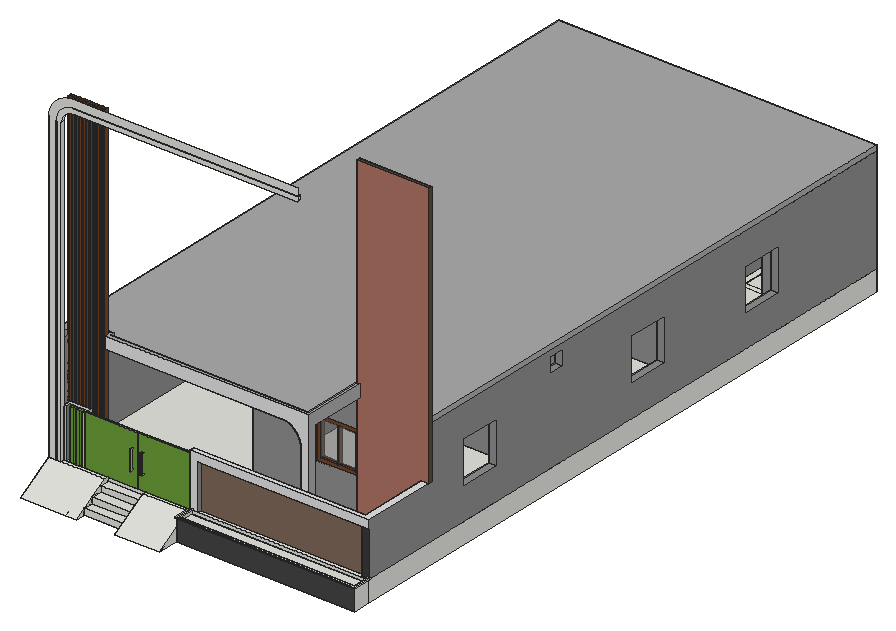
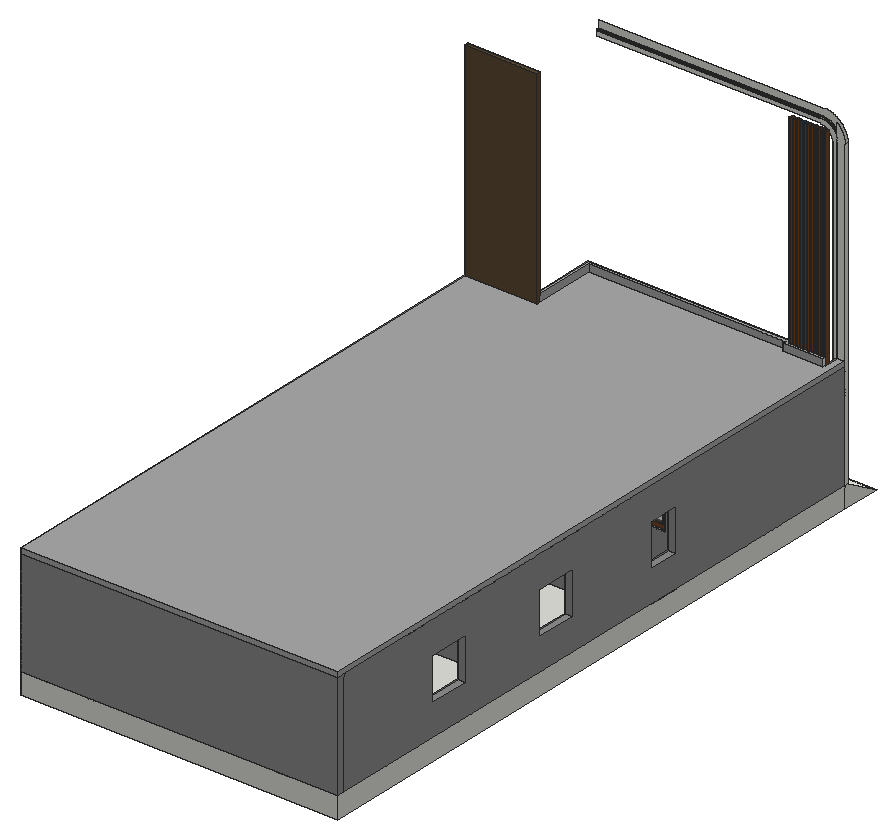
# SketchUp Ruby script. Lengths in inches.
U = 1.inch
M = Sketchup.active_model
def pt(a) = Geom::Point3d.new(a.map { |v| v * U })
def face(e, loops, mat)
  f = e.add_face(loops[0].map { |a| pt(a) })
  loops[1..].each { |l| e.add_face(l.map { |a| pt(a) }).erase! }
  f.material = f.back_material = mat if mat
  f
end
# faces: each face lists its corners as indices into pts; further lists are holes
def faces(e, pts, list, mat = nil) = list.each { |f| face(e, (f[0].is_a?(Array) ? f : [f]).map { |l| l.map { |i| pts[i] } }, mat) }
# xy, xz, yz: faces in a plane at the given z, y or x. An outline is a flat list of corners, or four numbers for a rectangle; further outlines are holes
def ring(l) = l.size == 4 ? [[l[0], l[1]], [l[2], l[1]], [l[2], l[3]], [l[0], l[3]]] : l.each_slice(2).to_a
def flat(e, list, mat, &to3) = list.each { |f| face(e, (f[0].is_a?(Array) ? f : [f]).map { |l| ring(l).map { |u, v| to3.(u, v) } }, mat) }
def xy(e, z, list, mat = nil) = flat(e, list, mat) { |x, y| [x, y, z] }
def xz(e, y, list, mat = nil) = flat(e, list, mat) { |x, z| [x, y, z] }
def yz(e, x, list, mat = nil) = flat(e, list, mat) { |y, z| [x, y, z] }
def lines(e, pts, list) = list.each { |a, b| e.add_line(pt(pts[a]), pt(pts[b])) }
# prism: a flat outline (further loops are holes) pulled along v
def prism(e, loops, v, mat = nil)
  f = face(e, loops, mat); d = Geom::Vector3d.new(v.map { |x| x * U })
  f.pushpull(f.normal.samedirection?(d) ? d.length : -d.length)
end
def box(e, o, s, mat = nil) = prism(e, [[o, [o[0] + s[0], o[1], o[2]], [o[0] + s[0], o[1] + s[1], o[2]], [o[0], o[1] + s[1], o[2]]]], [0, 0, s[2]], mat)
def at(x, y, z, deg = 0) = Geom::Transformation.translation(pt([x, y, z])) * Geom::Transformation.rotation(ORIGIN, Z_AXIS, deg.degrees)
def axes(o, x, y, z) = Geom::Transformation.new([*x, 0, *y, 0, *z, 0, *pt(o).to_a, 1])
def part(name) = M.definitions.add(name)
# library, detail: a bought-in or finely detailed component or shape, given as its bounding box
def library(name, o, s) = part(name).tap { |d| box(d.entities, o, s) }
def detail(e, o, s) = box(e.add_group.entities, o, s)
def put(e, d, t, mat = nil) = e.add_instance(d, t).tap { |i| i.material = mat if mat }
def group(e, t, mat = nil) = e.add_group.tap { |g| g.transformation = t; g.material = mat if mat }.entities
root = M.entities
M.materials.add("Material5_ met").color = [196, 146, 107]
M.materials.add("[Brick Rough Dark]").color = [94, 77, 53]
M.materials.add("[Color M01]").color = [226, 226, 226]
M.materials.add("[Color M03]").color = [170, 170, 170]
M.materials.add("[Color M04]").color = [142, 142, 142]
M.materials.add("[Color M07]").color = [58, 58, 58]
M.materials.add("[Granite Brown]").color = [126, 104, 91]
M.materials.add("[Granite Dark Gray]").color = [69, 68, 68]
M.materials.add("[Grass Dark Green]").color = [106, 157, 55]
M.materials.add("[Polished Concrete New]").color = [200, 200, 203]
M.materials.add("[Stone Flagstone Ashlar]").color = [175, 116, 102]
M.materials.add("[Translucent Glass Gray]").color = [128, 128, 128]
M.materials["[Translucent Glass Gray]"].alpha = 0.5
M.materials.add("[Wood Veneer 01]").color = [120, 70, 37]
M.materials.add("polished steel").color = [183, 187, 190]
M.materials.add("polished_ Blacktop Old 01").color = [132, 136, 139]
M.materials.add("steel").color = [179, 179, 179]
c1 = part("*U6")
p = [[-20,-17,0],[-20,23,0],[-18.25,23,0],[-18.25,-17,0],[20,-17,0],[19.92,-14.49,0],
  [19.68,-11.99,0],[19.29,-9.5,0],[18.74,-7.05,0],[18.04,-4.64,0],[17.19,-2.28,0],[16.19,0.03,0],
  [15.05,2.27,0],[13.77,4.43,0],[12.36,6.51,0],[10.82,8.5,0],[9.16,10.38,0],[7.38,12.16,0],
  [5.5,13.82,0],[3.51,15.36,0],[1.43,16.77,0],[-0.73,18.05,0],[-2.97,19.19,0],[-5.28,20.19,0],
  [-7.64,21.04,0],[-10.05,21.74,0],[-12.5,22.29,0],[-14.99,22.68,0],[-17.49,22.92,0],[-20,-23,0],
  [20,-23,0]]
lines(c1.entities,p,[[0,1],[1,2],[2,3],[3,0],[4,5],[5,6],[6,7],[7,8],[8,9],[9,10],[10,11],[11,12],
  [12,13],[13,14],[14,15],[15,16],[16,17],[17,18],[18,19],[19,20],[20,21],[21,22],[22,23],[23,24],
  [24,25],[25,26],[26,27],[27,28],[28,1],[0,29],[4,30]])
c2 = part("new block 03")
p = [[-4.5,18,0],[4.5,18,0],[4.5,-18,0],[-4.5,-18,0],[-1.33,-18,0],[-1.33,18,0],
  [1.57,18,0],[1.57,-18,0]]
lines(c2.entities,p,[[0,1],[1,2],[2,3],[3,0],[4,5],[5,6],[6,7]])
c3 = part("VENTILATOR")
p = [[-4.5,8.5,0],[4.5,8.5,0],[4.5,-8.5,0],[-4.5,-8.5,0],[0.58,8.5,0],[0.58,-8.5,0],
  [0,-8.5,0],[-1.15,-8.5,0],[-0.58,-8.5,0],[-0.58,8.5,0],[-1.15,8.5,0],[0,8.5,0]]
lines(c3.entities,p,[[0,1],[1,2],[2,3],[3,0],[4,5],[6,7],[8,9],[10,11]])
c4 = part("Bed - Queen")
p = [[22,23.6,0],[16.8,23.6,0],[22,38.8,0],[1.2,38.8,0],[1.2,25.6,0],[-1.2,38.8,0],
  [-1.2,25.6,0],[-22,38.8,0],[-22,25.6,0],[30,-40,0],[-30,-40,0],[-30,40,0],
  [14.8,23.2,0],[-30,23.2,0],[-30,25.6,0],[14.8,25.6,0],[30,40,0],[30,10.4,0],
  [14.8,10.4,0]]
lines(c4.entities,p,[[0,1],[2,0],[3,2],[4,3],[5,6],[7,5],[8,7],[9,10],[10,11],[12,13],[14,15],[11,16],
  [16,9],[17,15],[18,17],[15,18]])
c5 = library("*U4",[-21.75,-41.51,0],[21,28.01,0.01])
c6 = library("SINK",[-14.49,-22.42,0],[28.98,44.84,0.01])
c7 = part("new block 02")
p = [[-4.5,24,0],[4.5,24,0],[4.5,-24,0],[-4.5,-24,0],[-0.96,24,0],[-0.96,-24,0],
  [1.12,-24,0],[1.12,24,0]]
lines(c7.entities,p,[[0,1],[1,2],[2,3],[3,0],[4,5],[5,6],[6,7]])
c8 = library("PINTU 6 YA",[0,-0.6875,0],[35.83,8.07,80.71])
c9 = part("Group14\#1")
box(c9.entities,[324.26,626,0],[6,84,120])
c10 = part("Group16\#1")
box(c10.entities,[132.26,626,0],[6,84,120])
c11 = part("Group20\#1")
box(c11.entities,[233.26,464,0],[6,156,120])
c12 = part("Group25\#1")
xy(c12.entities,0,[[312.3125,242,312.3125,265.39,318.3125,265.39,318.3125,248,402.3125,248,402.3125,242],[312.3125,289.39,318.3125,296]])
xy(c12.entities,84,[[312.3125,265.39,318.3125,289.39]])
xy(c12.entities,120,[[312.3125,242,402.3125,242,402.3125,248,318.3125,248,318.3125,296,312.3125,296]])
xz(c12.entities,242,[[312.3125,0,402.3125,120]])
xz(c12.entities,248,[[318.3125,0,402.3125,120]])
xz(c12.entities,265.39,[[312.3125,0,318.3125,84]])
xz(c12.entities,289.39,[[312.3125,0,318.3125,84]])
xz(c12.entities,296,[[312.3125,0,318.3125,120]])
yz(c12.entities,312.3125,[[242,0,242,120,296,120,296,0,289.39,0,289.39,84,265.39,84,265.39,0]])
yz(c12.entities,318.3125,[[248,0,265.39,0,265.39,84,289.39,84,289.39,0,296,0,296,120,248,120]])
yz(c12.entities,402.3125,[[242,0,248,120]])
c13 = part("Group19\#1")
xy(c13.entities,0,[[-32.0625,-20.0625,-16.92,20.0625],[-15.73,-20.0625,-0.59,20.0625],[0.59,-20.0625,15.73,20.0625],[16.92,-20.0625,32.0625,20.0625]],"[Translucent Glass Gray]")
c14 = part("Group18\#1")
prism(c14.entities,[[[36,24,0],[36,-24,0],[-36,-24,0],[-36,24,0]],[[-15.73,20.0625,0],[-15.73,-20.0625,0],[-0.59,-20.0625,0],[-0.59,20.0625,0]],[[-32.0625,20.0625,0],[-32.0625,-20.0625,0],[-16.92,-20.0625,0],[-16.92,20.0625,0]],[[0.59,20.0625,0],[0.59,-20.0625,0],[15.73,-20.0625,0],[15.73,20.0625,0]],[[32.0625,20.0625,0],[16.92,20.0625,0],[16.92,-20.0625,0],[32.0625,-20.0625,0]]],[0,0,4],"[Wood Veneer 01]")
put(c14.entities,c13,at(0,0,2))
c15 = part("Group21\#2")
xy(c15.entities,0,[[-20.0625,-20.0625,-0.59,20.0625],[0.59,-20.0625,20.0625,20.0625]])
c16 = part("Group20\#3")
prism(c16.entities,[[[-24,24,0],[24,24,0],[24,-24,0],[-24,-24,0]],[[-20.0625,-20.0625,0],[-0.59,-20.0625,0],[-0.59,20.0625,0],[-20.0625,20.0625,0]],[[20.0625,20.0625,0],[0.59,20.0625,0],[0.59,-20.0625,0],[20.0625,-20.0625,0]]],[0,0,4],"[Wood Veneer 01]")
put(c16.entities,c15,at(0,0,2),"[Translucent Glass Gray]")
c17 = part("Group35\#1")
xy(c17.entities,0,[[-20.12,-20.0625,-0.59,20.0625],[0.59,-20.0625,20.12,20.0625]])
c18 = part("Group34\#2")
prism(c18.entities,[[[24.05,24,0],[24.05,-24,0],[-24.05,-24,0],[-24.05,24,0]],[[0.59,-20.0625,0],[20.12,-20.0625,0],[20.12,20.0625,0],[0.59,20.0625,0]],[[-20.12,-20.0625,0],[-0.59,-20.0625,0],[-0.59,20.0625,0],[-20.12,20.0625,0]]],[0,0,4],"[Wood Veneer 01]")
put(c18.entities,c17,at(0,0,2),"[Translucent Glass Gray]")
c19 = part("Union")
xy(c19.entities,0,[[273.03,12,282.03,21]])
xy(c19.entities,120,[[0,0,0,719,360.05,719,360.05,89,280.03,89,280.03,85,282.03,85,282.03,21,254.15,21,254.15,12,51,12,51,16,9,16,9,0]])
xy(c19.entities,126,[[0,0,9,0,9,20,55,20,55,16,278.03,16,278.03,85,280.03,85,280.03,89,360.05,89,360.05,719,0,719]])
xy(c19.entities,134,[[51,12,282.03,12,282.03,85,278.03,85,278.03,16,55,16,55,20,9,20,9,16,51,16]])
xz(c19.entities,0,[[0,120,9,126]])
xz(c19.entities,12,[[273.03,0,282.03,0,282.03,134,51,134,51,120,254.15,120,254.78,119.94,255.41,119.81,256.03,119.65,256.64,119.48,257.25,119.29,257.85,119.09,258.45,118.87,259.04,118.63,259.625,118.375,260.2,118.1,260.77,117.82,261.33,117.51,261.88,117.19,262.43,116.86,262.96,116.51,263.48,116.15,264,115.77,264.5,115.38,264.99,114.97,265.47,114.55,265.9375,114.12,266.39,113.68,266.84,113.22,267.27,112.75,268.09,111.77,268.48,111.27,268.85,110.75,269.21,110.23,269.56,109.69,269.89,109.14,270.2,108.59,270.5,108.03,270.78,107.46,271.05,106.88,271.3,106.29,271.54,105.7,271.76,105.1,271.96,104.5,272.14,103.89,272.31,103.27,272.46,102.65,272.59,102.03,272.71,101.4,272.8,100.77,272.88,100.14,272.95,99.51,272.99,98.87,273.02,98.23,273.03,97.6]],"[Color M01]")
xz(c19.entities,16,[[55,126,278.03,134]])
xz(c19.entities,16,[[9,120,51,126],[9,126,51,134]],"[Color M01]")
xz(c19.entities,20,[[9,126,55,134]])
xz(c19.entities,21,[[273.03,0,273.03,97.6,273.02,98.23,272.99,98.87,272.95,99.51,272.88,100.14,272.8,100.77,272.71,101.4,272.59,102.03,272.46,102.65,272.31,103.27,272.14,103.89,271.96,104.5,271.76,105.1,271.54,105.7,271.3,106.29,271.05,106.88,270.78,107.46,270.5,108.03,270.2,108.59,269.89,109.14,269.56,109.69,269.21,110.23,268.85,110.75,268.48,111.27,268.09,111.77,267.27,112.75,266.84,113.22,266.39,113.68,265.9375,114.12,265.47,114.55,264.99,114.97,264.5,115.38,264,115.77,263.48,116.15,262.96,116.51,262.43,116.86,261.88,117.19,261.33,117.51,260.77,117.82,260.2,118.1,259.625,118.375,259.04,118.63,258.45,118.87,257.85,119.09,257.25,119.29,256.64,119.48,256.03,119.65,255.41,119.81,254.78,119.94,254.15,120,282.03,120,282.03,0]])
xz(c19.entities,85,[[280.03,120,282.03,126],[278.03,126,282.03,134]])
xz(c19.entities,89,[[280.03,120,360.05,126]])
xz(c19.entities,719,[[0,120,360.05,126]])
yz(c19.entities,0,[[0,120,719,126]])
yz(c19.entities,9,[[0,120,16,126]])
yz(c19.entities,9,[[16,126,20,134]],"[Color M01]")
yz(c19.entities,51,[[12,120,16,134]],"[Color M01]")
yz(c19.entities,55,[[16,126,20,134]])
yz(c19.entities,273.03,[[12,0,21,97.6]])
yz(c19.entities,278.03,[[16,126,85,134]])
yz(c19.entities,280.03,[[85,120,89,126]])
yz(c19.entities,282.03,[[12,0,21,0,21,120,85,120,85,134,12,134]])
yz(c19.entities,360.05,[[89,120,719,126]])
p = [[273.03,12,97.6],[273.02,12,98.23],[273.02,21,98.23],[273.03,21,97.6],[272.99,12,98.87],[272.99,21,98.87],
  [272.95,12,99.51],[272.95,21,99.51],[272.88,12,100.14],[272.88,21,100.14],[272.8,12,100.77],[272.8,21,100.77],
  [272.71,12,101.4],[272.71,21,101.4],[272.59,12,102.03],[272.59,21,102.03],[272.46,12,102.65],[272.46,21,102.65],
  [272.31,12,103.27],[272.31,21,103.27],[272.14,12,103.89],[272.14,21,103.89],[271.96,12,104.5],[271.96,21,104.5],
  [271.76,12,105.1],[271.76,21,105.1],[271.54,12,105.7],[271.54,21,105.7],[271.3,12,106.29],[271.3,21,106.29],
  [271.05,12,106.88],[271.05,21,106.88],[270.78,12,107.46],[270.78,21,107.46],[270.5,12,108.03],[270.5,21,108.03],
  [270.2,12,108.59],[270.2,21,108.59],[269.89,12,109.14],[269.89,21,109.14],[269.56,12,109.69],[269.56,21,109.69],
  [269.21,12,110.23],[269.21,21,110.23],[268.85,12,110.75],[268.85,21,110.75],[268.48,12,111.27],[268.48,21,111.27],
  [268.09,12,111.77],[268.09,21,111.77],[267.68,12,112.26],[267.68,21,112.26],[267.27,12,112.75],[267.27,21,112.75],
  [266.84,12,113.22],[266.84,21,113.22],[266.39,12,113.68],[266.39,21,113.68],[265.9375,12,114.12],[265.9375,21,114.12],
  [265.47,12,114.55],[265.47,21,114.55],[264.99,12,114.97],[264.99,21,114.97],[264.5,12,115.38],[264.5,21,115.38],
  [264,12,115.77],[264,21,115.77],[263.48,12,116.15],[263.48,21,116.15],[262.96,12,116.51],[262.96,21,116.51],
  [262.43,12,116.86],[262.43,21,116.86],[261.88,12,117.19],[261.88,21,117.19],[261.33,12,117.51],[261.33,21,117.51],
  [260.77,12,117.82],[260.77,21,117.82],[260.2,12,118.1],[260.2,21,118.1],[259.625,12,118.375],[259.625,21,118.375],
  [259.04,12,118.63],[259.04,21,118.63],[258.45,12,118.87],[258.45,21,118.87],[257.85,12,119.09],[257.85,21,119.09],
  [257.25,12,119.29],[257.25,21,119.29],[256.64,12,119.48],[256.64,21,119.48],[256.03,12,119.65],[256.03,21,119.65],
  [255.41,12,119.81],[255.41,21,119.81],[254.78,12,119.94],[254.78,21,119.94],[254.15,12,120],[254.15,21,120]]
faces(c19.entities,p,[[0,1,2,3],[1,4,5,2],[4,6,7,5],[6,8,9,7],[8,10,11,9],[10,12,13,11],[12,14,15,13],[14,16,17,15],
  [16,18,19,17],[18,20,21,19],[20,22,23,21],[22,24,25,23],[24,26,27,25],[26,28,29,27],[28,30,31,29],[30,32,33,31],
  [32,34,35,33],[34,36,37,35],[36,38,39,37],[38,40,41,39],[40,42,43,41],[42,44,45,43],[44,46,47,45],[46,48,49,47],
  [48,50,51,49],[50,52,53,51],[52,54,55,53],[54,56,57,55],[56,58,59,57],[58,60,61,59],[60,62,63,61],[62,64,65,63],
  [64,66,67,65],[66,68,69,67],[68,70,71,69],[70,72,73,71],[72,74,75,73],[74,76,77,75],[76,78,79,77],[78,80,81,79],
  [80,82,83,81],[82,84,85,83],[84,86,87,85],[86,88,89,87],[88,90,91,89],[90,92,93,91],[92,94,95,93],[94,96,97,95],
  [96,98,99,97],[98,100,101,99]])
c20 = part("faewg")
xy(c20.entities,0,[[0,-3,2,0]])
xy(c20.entities,1,[[0,-2,2,0]])
xy(c20.entities,23,[[0,-2,2,0]])
xy(c20.entities,24,[[0,-3,2,0]])
xz(c20.entities,-3,[[0,0,2,24]],"polished steel")
xz(c20.entities,-2,[[0,1,2,23]])
xz(c20.entities,0,[[0,0,2,1],[0,23,2,24]])
yz(c20.entities,0,[[-3,0,-3,24,0,24,0,23,-2,23,-2,1,0,1,0,0]])
yz(c20.entities,2,[[-3,0,0,0,0,1,-2,1,-2,23,0,23,0,24,-3,24]])
c21 = part("reg")
xy(c21.entities,0,[[-8.95,3,59.93,5]])
xy(c21.entities,18,[[51.93,0,53.93,3]],"steel")
xy(c21.entities,19,[[51.93,1,53.93,3]],"steel")
xy(c21.entities,41,[[51.93,1,53.93,3]],"steel")
xy(c21.entities,42,[[51.93,0,53.93,3]],"steel")
xy(c21.entities,61,[[-8.95,3,59.93,5]])
xz(c21.entities,0,[[51.93,18,53.93,42]],"polished steel")
xz(c21.entities,1,[[51.93,19,53.93,41]],"steel")
xz(c21.entities,3,[[[-8.95,0,59.93,61],[51.93,18,53.93,19],[51.93,41,53.93,42]]])
xz(c21.entities,3,[[51.93,18,53.93,19],[51.93,41,53.93,42]],"steel")
xz(c21.entities,5,[[-8.95,0,59.93,61]])
yz(c21.entities,-8.95,[[3,0,5,61]])
yz(c21.entities,51.93,[[0,18,0,42,3,42,3,41,1,41,1,19,3,19,3,18]],"steel")
yz(c21.entities,53.93,[[0,18,3,18,3,19,1,19,1,41,3,41,3,42,0,42]],"steel")
yz(c21.entities,59.93,[[3,0,5,61]])
put(c21.entities,c20,axes([51.93,5.4375,42],[1,0,0],[0,-1,0],[0,0,-1]),"steel")
c22 = part("gbsrtn")
put(c22.entities,c21,at(402.95,-3,0))
put(c22.entities,c21,axes([522.82,-3,0],[-1,0,0],[0,1,0],[0,0,1]))
g1 = group(c22.entities,at(366,9,0),"polished_ Blacktop Old 01")
xy(g1,0,[[0,-9,0,0,28,0,28,-9,24,-9,24,-5,4,-5,4,-9]])
xy(g1,60,[[0,-9,4,-9,4,-5,24,-5,24,-9,28,-9,28,0,0,0]],"[Polished Concrete New]")
xz(g1,-9,[[0,0,4,60],[24,0,28,60]],"[Polished Concrete New]")
xz(g1,-5,[[4,0,24,60]],"Material5_ met")
xz(g1,0,[[0,0,28,60]])
yz(g1,0,[[-9,0,0,60]],"[Polished Concrete New]")
yz(g1,4,[[-9,0,-5,60]],"polished_ Blacktop Old 01")
yz(g1,24,[[-9,0,-5,60]],"polished_ Blacktop Old 01")
yz(g1,28,[[-9,0,0,60]],"[Polished Concrete New]")
g2 = group(c22.entities,at(12.5,0,0))
prism(g2,[[[365.99,4,0],[365.99,4,4],[365.99,4,56],[365.99,4,60],[365.99,0,60],[365.99,0,0]]],[-5,0,0])
prism(g2,[[[374.53,4,0],[374.53,4,4],[374.53,4,56],[374.53,4,60],[374.53,0,60],[374.53,0,0]]],[-5,0,0])
c23 = part("main gate")
put(c23.entities,c22,at(100.96,59.79,1),"[Grass Dark Green]")
xy(root,0,[[0,40.1875,0,44.1875,9,44.1875,9,43.1875,8.11,43.1875,8.11,40.1875],[9,40.1875,14,44.1875]])
xz(root,40.1875,[[0,0,8.11,0,8.11,344.13,8.12,344.75,8.14,345.37,8.19,345.99,8.26,346.61,8.35,347.22,8.46,347.83,8.58,348.44,8.73,349.05,8.89,349.64,9.07,350.24,9.27,350.83,9.49,351.41,9.73,351.98,9.99,352.55,10.26,353.1,10.55,353.65,10.86,354.19,11.18,354.72,11.52,355.24,11.88,355.75,12.25,356.24,12.64,356.73,13.04,357.2,13.46,357.66,13.89,358.11,14.34,358.54,14.8,358.96,15.27,359.36,15.76,359.75,16.25,360.12,16.76,360.48,17.28,360.82,17.81,361.14,18.35,361.45,18.9,361.74,19.45,362.01,20.02,362.27,20.59,362.51,21.17,362.73,21.76,362.93,22.36,363.11,22.95,363.27,23.56,363.42,24.17,363.54,24.78,363.65,25.39,363.74,26.01,363.81,26.63,363.86,27.25,363.88,27.87,363.89,282.03,363.89,282.03,372,25.95,372,25.24,371.94,24.37,371.85,23.5,371.72,22.63,371.57,21.77,371.4,20.92,371.19,20.07,370.96,19.24,370.7,18.41,370.42,17.58,370.11,16.77,369.77,15.97,369.41,15.1875,369.02,14.41,368.61,13.65,368.18,12.9,367.72,12.17,367.24,11.45,366.73,10.75,366.21,10.0625,365.66,9.39,365.09,8.74,364.5,8.11,363.89,7.5,363.26,6.91,362.61,6.34,361.9375,5.79,361.25,5.27,360.55,4.76,359.83,4.28,359.1,3.82,358.35,3.39,357.59,2.98,356.8125,2.59,356.03,2.23,355.23,1.89,354.42,1.58,353.59,1.3,352.76,1.04,351.93,0.81,351.08,0.6,350.23,0.43,349.37,0.28,348.5,0.15,347.63,0.06,346.76,0,346.05],[9,0,14,0,14,344.13,14.01,344.57,14.03,345,14.0625,345.4375,14.11,345.87,14.17,346.3,14.33,347.16,14.4375,347.58,14.55,348,14.68,348.42,14.82,348.83,14.97,349.24,15.14,349.64,15.32,350.04,15.51,350.43,15.72,350.8125,15.93,351.19,16.16,351.5625,16.4,351.93,16.65,352.28,16.91,352.63,17.18,352.97,17.47,353.3,17.76,353.625,18.0625,353.9375,18.375,354.24,18.7,354.53,19.03,354.82,19.37,355.09,19.72,355.35,20.07,355.6,20.4375,355.84,20.81,356.07,21.1875,356.28,21.57,356.49,21.96,356.68,22.36,356.86,22.76,357.03,23.17,357.18,23.58,357.32,24,357.45,24.42,357.5625,24.84,357.67,25.7,357.83,26.13,357.89,26.5625,357.9375,27,357.97,27.43,357.99,27.87,358,282.03,358,282.03,363,27.87,363,27.28,362.99,26.68,362.96,26.09,362.92,25.5,362.85,24.92,362.77,24.33,362.67,23.75,362.55,23.18,362.41,22.6,362.25,22.04,362.08,21.48,361.88,20.92,361.67,20.375,361.45,19.83,361.2,19.3,360.94,18.78,360.67,18.26,360.37,17.76,360.0625,17.26,359.74,16.78,359.4,16.3,359.04,15.84,358.67,15.39,358.28,14.95,357.89,14.11,357.05,13.72,356.61,13.33,356.16,12.96,355.7,12.6,355.22,12.26,354.74,11.9375,354.24,11.63,353.74,11.33,353.22,11.06,352.7,10.8,352.17,10.55,351.625,10.33,351.08,10.12,350.52,9.92,349.96,9.75,349.4,9.59,348.82,9.45,348.25,9.33,347.67,9.23,347.08,9.15,346.5,9.08,345.91,9.04,345.32,9.01,344.72,9,344.13]])
xz(root,43.1875,[[8.11,0,9,0,9,344.13,9.01,344.72,9.04,345.32,9.08,345.91,9.15,346.5,9.23,347.08,9.33,347.67,9.45,348.25,9.59,348.82,9.75,349.4,9.92,349.96,10.12,350.52,10.33,351.08,10.55,351.625,10.8,352.17,11.06,352.7,11.33,353.22,11.63,353.74,11.9375,354.24,12.26,354.74,12.6,355.22,12.96,355.7,13.33,356.16,13.72,356.61,14.11,357.05,14.95,357.89,15.39,358.28,15.84,358.67,16.3,359.04,16.78,359.4,17.26,359.74,17.76,360.0625,18.26,360.37,18.78,360.67,19.3,360.94,19.83,361.2,20.375,361.45,20.92,361.67,21.48,361.88,22.04,362.08,22.6,362.25,23.18,362.41,23.75,362.55,24.33,362.67,24.92,362.77,25.5,362.85,26.09,362.92,26.68,362.96,27.28,362.99,27.87,363,282.03,363,282.03,363.89,27.87,363.89,27.25,363.88,26.63,363.86,26.01,363.81,25.39,363.74,24.78,363.65,24.17,363.54,23.56,363.42,22.95,363.27,22.36,363.11,21.76,362.93,21.17,362.73,20.59,362.51,20.02,362.27,19.45,362.01,18.9,361.74,18.35,361.45,17.81,361.14,17.28,360.82,16.76,360.48,16.25,360.12,15.76,359.75,15.27,359.36,14.8,358.96,14.34,358.54,13.89,358.11,13.46,357.66,13.04,357.2,12.64,356.73,12.25,356.24,11.88,355.75,11.52,355.24,11.18,354.72,10.86,354.19,10.55,353.65,10.26,353.1,9.99,352.55,9.73,351.98,9.49,351.41,9.27,350.83,9.07,350.24,8.89,349.64,8.73,349.05,8.58,348.44,8.46,347.83,8.35,347.22,8.26,346.61,8.19,345.99,8.14,345.37,8.12,344.75,8.11,344.13]])
xz(root,44.1875,[[0,0,0,346.05,0.06,346.76,0.15,347.63,0.28,348.5,0.43,349.37,0.6,350.23,0.81,351.08,1.04,351.93,1.3,352.76,1.58,353.59,1.89,354.42,2.23,355.23,2.59,356.03,2.98,356.8125,3.39,357.59,3.82,358.35,4.28,359.1,4.76,359.83,5.27,360.55,5.79,361.25,6.34,361.9375,6.91,362.61,7.5,363.26,8.11,363.89,8.74,364.5,9,364.73,9,0],[9,0,9,344.13,9.01,344.72,9.02,345.02,9.04,345.32,9.08,345.91,9.15,346.5,9.23,347.08,9.33,347.67,9.45,348.25,9.59,348.82,9.75,349.4,9.92,349.96,10.12,350.52,10.33,351.08,10.55,351.625,10.8,352.17,11.06,352.7,11.33,353.22,11.63,353.74,11.9375,354.24,12.26,354.74,12.6,355.22,12.96,355.7,13.33,356.16,13.72,356.61,14.11,357.05,14.95,357.89,15.39,358.28,15.84,358.67,16.3,359.04,16.78,359.4,17.26,359.74,17.76,360.0625,18.26,360.37,18.78,360.67,19.3,360.94,19.83,361.2,20.375,361.45,20.92,361.67,21.48,361.88,22.04,362.08,22.6,362.25,23.18,362.41,23.75,362.55,24.33,362.67,24.92,362.77,25.5,362.85,26.09,362.92,26.68,362.96,27.28,362.99,27.87,363,282.03,363,282.03,358,27.87,358,27.43,357.99,27,357.97,26.5625,357.9375,26.13,357.89,25.7,357.83,24.84,357.67,24.42,357.5625,24,357.45,23.58,357.32,23.17,357.18,22.76,357.03,22.36,356.86,21.96,356.68,21.57,356.49,21.1875,356.28,20.81,356.07,20.4375,355.84,20.07,355.6,19.72,355.35,19.37,355.09,19.03,354.82,18.7,354.53,18.375,354.24,18.0625,353.9375,17.76,353.625,17.47,353.3,17.18,352.97,16.91,352.63,16.65,352.28,16.4,351.93,16.16,351.5625,15.93,351.19,15.72,350.8125,15.51,350.43,15.32,350.04,15.14,349.64,14.97,349.24,14.82,348.83,14.68,348.42,14.55,348,14.4375,347.58,14.33,347.16,14.17,346.3,14.11,345.87,14.0625,345.4375,14.03,345,14.01,344.57,14,344.13,14,0]])
yz(root,0,[[40.1875,0,44.1875,346.05]])
yz(root,8.11,[[40.1875,0,43.1875,344.13]])
yz(root,9,[[40.1875,0,43.1875,344.13],[43.1875,0,44.1875,344.13]])
yz(root,14,[[40.1875,0,44.1875,344.13]])
p = [[106.59,40.1875,0],[106.59,0,-24]]
lines(root,p,[[0,1]])
g3 = group(root,at(157,44.1875,-24))
g4 = group(g3,at(0,-20,0))
xy(g4,0,[[1,0,203.05,20]])
xy(g4,19.75,[[2,2,201.05,20]])
xy(g4,24,[[1,0,203.05,0,203.05,18,201.05,18,201.05,2,2,2,2,20,1,20],[201.05,18,203.05,20]])
xz(g4,0,[[1,0,203.05,24]],"[Granite Dark Gray]")
xz(g4,2,[[2,19.75,201.05,24]])
xz(g4,20,[[1,0,1,24,2,24,2,19.75,201.05,19.75,201.05,24,203.05,24,203.05,0]])
yz(g4,1,[[0,0,20,24]])
yz(g4,2,[[2,19.75,20,24]])
yz(g4,201.05,[[2,19.75,20,24]])
yz(g4,203.05,[[0,0,20,24]])
g5 = group(root,at(0,44.1875,-24))
xy(g5,0,[[63.66,-33.1,63.66,0,0,0,0,719,360.05,719,360.05,0,106.59,0,106.59,-33.1]])
xy(g5,6.83,[[63.66,-33.1,106.59,-22.47]])
xy(g5,13.125,[[63.66,-22.47,106.59,-9.875]])
xy(g5,19.6,[[63.66,-9.875,106.59,0]])
xy(g5,24,[[0,0,360.05,719]])
xz(g5,-33.1,[[63.66,0,106.59,6.83]])
xz(g5,-22.47,[[63.66,6.83,106.59,13.125]])
xz(g5,-9.875,[[63.66,13.125,106.59,19.6]])
xz(g5,0,[[0,0,63.66,24],[106.59,0,360.05,24],[63.66,19.6,106.59,24]])
xz(g5,719,[[0,0,360.05,24]])
yz(g5,0,[[0,0,719,24]])
yz(g5,63.66,[[-33.1,0,-33.1,6.83,-22.47,6.83,-22.47,8,0,8,0,0],[-22.47,8,-22.47,13.125,-15.3125,13.125,-15.3125,9.9375,0,9.9375,0,8],[-15.3125,9.9375,-15.3125,13.125,-9.875,13.125,-9.875,19.6,0,19.6,0,9.9375]])
yz(g5,106.59,[[-33.1,0,0,0,0,8,-22.47,8,-22.47,6.83,-33.1,6.83],[-22.47,8,0,8,0,9.9375,-15.3125,9.9375,-15.3125,13.125,-22.47,13.125],[-15.3125,9.9375,0,9.9375,0,19.6,-9.875,19.6,-9.875,13.125,-15.3125,13.125]])
yz(g5,360.05,[[0,0,719,24]])
g6 = group(root,at(0,0,-24))
xy(g6,0,[[106.59,0,158,44.1875]])
xy(g6,24,[[106.59,40.1875,158,44.1875]])
xz(g6,44.1875,[[106.59,0,158,24]])
yz(g6,106.59,[[0,0,40.1875,24,44.1875,24,44.1875,0]])
yz(g6,158,[[0,0,44.1875,0,44.1875,24,40.1875,24]])
p = [[106.59,40.1875,24],[106.59,0,0],[158,0,0],[158,40.1875,24],[157,44.1875,24]]
faces(g6,p,[[0,1,2,3]])
lines(g6,p,[[4,2]])
g7 = group(root,at(-106.59,0,-24))
xy(g7,0,[[106.59,0,170.25,44.1875]])
xy(g7,24,[[106.59,40.1875,170.25,44.1875]])
xz(g7,44.1875,[[106.59,0,170.25,24]])
yz(g7,106.59,[[0,0,40.1875,24,44.1875,24,44.1875,0]])
yz(g7,170.25,[[0,0,44.1875,0,44.1875,24,40.1875,24]])
p = [[106.59,40.1875,24],[106.59,0,0],[158,0,0],[170.25,0,0],[170.25,40.1875,24],[157,44.1875,24]]
faces(g7,p,[[0,1,2,3,4]])
lines(g7,p,[[5,2]])
g8 = group(root,at(156,23.1875,0))
prism(g8,[[[4,3,0],[202.05,3,0],[202.05,22,0],[205.05,22,0],[205.05,0,0],[1,0,0],[1,21,0],[4,21,0]]],[0,0,1])
g9 = group(root,at(157,24.1875,0))
xy(g9,0,[[0,0,203.05,0,203.05,18,201.05,18,201.05,2,2,2,2,20,0,20]])
g10 = group(root,at(-51.08,44.1875,0),"[Color M04]")
xy(g10,0,[[51.08,0,60.08,239.47],[208.08,0,208.08,6,402.13,6,402.13,371.28,411.13,371.28,411.13,1,402.13,1,402.13,4,217.08,4,217.08,0],[208.08,89,208.08,106,217.08,106,217.08,98,281.11,98,281.11,89],[281.11,89,329.11,92.38],[329.11,89,402.13,98],
  [281.11,92.38,329.11,94.46],[281.11,94.46,329.11,98],[217.08,98,217.14,106.25],[208.08,106,217.08,106.25],[208.08,135.66,208.08,136,217.08,135.66],
  [217.08,135.66,208.08,136,208.08,146.08,217.08,146.08],[208.08,146.08,211.62,146.14],[211.62,146.08,213.7,146.14],[213.7,146.08,217.08,146.14],[208.08,146.14,211.62,194.08],
  [211.62,146.14,213.7,194.08],[213.7,146.14,217.08,194.08],[208.08,194.08,217.08,206],[60.08,206,174.57,215],[204.57,206,208.08,215],
  [208.08,206,217.08,302],[51.08,239.47,60.08,385.56],[60.08,293,174.15,302],[276.13,296,402.13,302],[276.13,302,282.13,317.31],
  [276.13,347.31,282.13,458],[60.08,458,197.65,464],[227.65,458,243.25,464],[273.25,458,402.13,464],[402.13,532.1875,402.13,710,324.08,710,324.08,719,411.13,719,411.13,532.1875],
  [51.08,537.75,51.08,719,138.08,719,138.08,710,60.08,710,60.08,537.75],[60.08,620,103.1,626],[127.1,620,143.64,626],[173.64,620,286.625,626],[316.625,620,336.8,626],
  [360.8,620,402.13,626]])
xy(g10,36,[[281.11,89,329.11,98],[402.13,133.01,411.13,181.01],[208.08,146.14,217.08,194.25],[84.08,206,156.08,215],[51.08,239.47,60.08,275.35],
  [402.13,371.28,411.13,419.28],[51.08,385.56,60.08,433.56],[402.13,532.1875,411.13,580.1875],[51.08,537.75,60.08,585.75]])
xy(g10,51,[[217.08,0,402.13,4],[402.13,0,411.13,1]])
xy(g10,60,[[208.08,0,411.13,0,411.13,89,402.13,89,402.13,6,208.08,6]],"[Color M01]")
xy(g10,84,[[281.11,89,329.11,98],[208.08,106.25,217.08,135.66],[402.13,133.01,411.13,181.01],[208.08,146.14,217.08,194.25],[84.08,206,156.08,215],
  [174.57,206,204.57,215],[51.08,239.47,60.08,275.35],[174.15,293,208.08,302],[276.13,317.31,282.13,347.31],[402.13,371.28,411.13,419.28],
  [51.08,385.56,60.08,433.56],[197.65,458,227.65,464],[243.25,458,273.25,464],[402.13,532.1875,411.13,580.1875],[51.08,537.75,60.08,585.75],
  [103.1,620,127.1,626],[143.64,620,173.64,626],[286.625,620,316.625,626],[336.8,620,360.8,626]])
xy(g10,96,[[402.13,256.23,411.13,274.23]])
xy(g10,114,[[402.13,256.23,411.13,274.23]])
xy(g10,120,[[51.08,0,60.08,710],[208.08,89,411.13,89,411.13,719,51.08,719,51.08,710,402.13,710,402.13,98,217.14,98,217.14,106.25,217.08,106.25,217.08,302,60.08,302,60.08,293,208.08,293,208.08,215,60.08,215,60.08,206,208.08,206],[276.13,296,402.13,296,402.13,302,282.13,302,282.13,458,276.13,458],[60.08,458,402.13,464],[60.08,620,402.13,626]])
xz(g10,0,[[51.08,0,60.08,120]])
xz(g10,0,[[208.08,0,217.08,0,217.08,51,411.13,51,411.13,60,208.08,60]],"[Color M01]")
xz(g10,1,[[402.13,0,411.13,51]],"[Color M07]")
xz(g10,4,[[217.08,0,402.13,51]],"[Granite Brown]")
xz(g10,6,[[208.08,0,402.13,60]])
xz(g10,89,[[[208.08,0,402.13,0,402.13,60,411.13,60,411.13,120,208.08,120],[281.11,36,329.11,84]]])
xz(g10,98,[[[217.14,0,402.13,120],[281.11,36,329.11,84]]])
xz(g10,106.25,[[208.08,0,208.08,84,217.08,84,217.08,120,217.14,120,217.14,0]])
xz(g10,133.01,[[402.13,36,411.13,84]])
xz(g10,135.66,[[208.08,0,217.08,84]])
xz(g10,146.14,[[208.08,36,217.08,84]])
xz(g10,181.01,[[402.13,36,411.13,84]])
xz(g10,194.25,[[208.08,36,217.08,84]])
xz(g10,206,[[[60.08,0,174.57,0,174.57,84,204.57,84,204.57,0,208.08,0,208.08,120,60.08,120],[84.08,36,156.08,84]]])
xz(g10,215,[[[60.08,0,60.08,120,208.08,120,208.08,0,204.57,0,204.57,84,174.57,84,174.57,0],[84.08,36,156.08,84]]])
xz(g10,239.47,[[51.08,36,60.08,84]])
xz(g10,256.23,[[402.13,96,411.13,114]])
xz(g10,274.23,[[402.13,96,411.13,114]])
xz(g10,275.35,[[51.08,36,60.08,84]])
xz(g10,293,[[60.08,0,174.15,0,174.15,84,208.08,84,208.08,120,60.08,120]])
xz(g10,296,[[276.13,0,402.13,120]])
xz(g10,302,[[60.08,0,60.08,120,217.08,120,217.08,0,208.08,0,208.08,84,174.15,84,174.15,0],[282.13,0,402.13,120]])
xz(g10,317.31,[[276.13,0,282.13,84]])
xz(g10,347.31,[[276.13,0,282.13,84]])
xz(g10,371.28,[[402.13,36,411.13,84]])
xz(g10,385.56,[[51.08,36,60.08,84]])
xz(g10,419.28,[[402.13,36,411.13,84]])
xz(g10,433.56,[[51.08,36,60.08,84]])
xz(g10,458,[[60.08,0,197.65,0,197.65,84,227.65,84,227.65,0,243.25,0,243.25,84,273.25,84,273.25,0,276.13,0,276.13,120,60.08,120],[276.13,0,282.13,120],[282.13,0,402.13,120]])
xz(g10,464,[[60.08,0,60.08,120,402.13,120,402.13,0,273.25,0,273.25,84,243.25,84,243.25,0,227.65,0,227.65,84,197.65,84,197.65,0]])
xz(g10,532.1875,[[402.13,36,411.13,84]])
xz(g10,537.75,[[51.08,36,60.08,84]])
xz(g10,580.1875,[[402.13,36,411.13,84]])
xz(g10,585.75,[[51.08,36,60.08,84]])
xz(g10,620,[[60.08,0,103.1,0,103.1,84,127.1,84,127.1,0,143.64,0,143.64,84,173.64,84,173.64,0,286.625,0,286.625,84,316.625,84,316.625,0,336.8,0,336.8,84,360.8,84,360.8,0,402.13,0,402.13,120,60.08,120]])
xz(g10,626,[[60.08,0,60.08,120,127.1,120,127.1,84,103.1,84,103.1,0],[127.1,0,143.64,120],[173.64,0,173.64,84,143.64,84,143.64,120,402.13,120,402.13,0,360.8,0,360.8,84,336.8,84,336.8,0,316.625,0,316.625,84,286.625,84,286.625,0]])
xz(g10,710,[[60.08,0,402.13,120]])
xz(g10,719,[[51.08,0,411.13,120]])
yz(g10,51.08,[[[0,0,710,120],[537.75,36,585.75,84],[385.56,36,433.56,84],[239.47,36,275.35,84]],[710,0,719,120]])
yz(g10,60.08,[[0,0,206,120],[206,0,215,120],[[215,0,293,120],[239.47,36,275.35,84]],[293,0,302,120],[[302,0,458,120],[385.56,36,433.56,84]],
  [458,0,464,120],[[464,0,620,120],[537.75,36,585.75,84]],[620,0,626,120],[626,0,710,120]])
yz(g10,84.08,[[206,36,215,84]])
yz(g10,103.1,[[620,0,626,84]])
yz(g10,127.1,[[620,0,626,84]])
yz(g10,143.64,[[620,0,626,84]])
yz(g10,156.08,[[206,36,215,84]])
yz(g10,173.64,[[620,0,626,84]])
yz(g10,174.15,[[293,0,302,84]])
yz(g10,174.57,[[206,0,215,84]])
yz(g10,197.65,[[458,0,464,84]])
yz(g10,204.57,[[206,0,215,84]])
yz(g10,208.08,[[[89,0,89,120,206,120,206,0,135.66,0,135.66,84,106.25,84,106.25,0],[146.14,36,194.25,84]],[215,0,215,120,293,120,293,84,302,84,302,0]])
yz(g10,208.08,[[0,0,6,60]],"[Color M01]")
yz(g10,217.08,[[0,0,4,51],[[135.66,0,302,0,302,120,106.25,120,106.25,84,135.66,84],[146.14,36,194.25,84]]])
yz(g10,217.14,[[98,0,106.25,120]])
yz(g10,227.65,[[458,0,464,84]])
yz(g10,243.25,[[458,0,464,84]])
yz(g10,273.25,[[458,0,464,84]])
yz(g10,276.13,[[296,0,296,120,458,120,458,0,347.31,0,347.31,84,317.31,84,317.31,0]])
yz(g10,281.11,[[89,36,98,84]])
yz(g10,282.13,[[302,0,317.31,0,317.31,84,347.31,84,347.31,0,458,0,458,120,302,120]])
yz(g10,286.625,[[620,0,626,84]])
yz(g10,316.625,[[620,0,626,84]])
yz(g10,329.11,[[89,36,98,84]])
yz(g10,336.8,[[620,0,626,84]])
yz(g10,360.8,[[620,0,626,84]])
yz(g10,402.13,[[1,0,4,51],[6,0,89,60],[[98,0,296,120],[133.01,36,181.01,84],[256.23,96,274.23,114]],[296,0,302,120],[302,0,371.28,120],
  [371.28,0,371.28,36,419.28,36,419.28,84,371.28,84,371.28,120,458,120,458,0],[458,0,464,120],[[464,0,620,120],[532.1875,36,580.1875,84]],[620,0,626,120],[626,0,710,120]])
yz(g10,411.13,[[[1,0,719,0,719,120,89,120,89,60,0,60,0,51,1,51],[532.1875,36,580.1875,84],[133.01,36,181.01,84],[371.28,36,419.28,84],[256.23,96,274.23,114]]])
p = [[62.99,709.53,0],[62.83,709.52,0],[62.67,709.49,0],[62.52,709.46,0],[62.37,709.41,0],[62.22,709.36,0],
  [62.08,709.29,0],[61.94,709.22,0],[61.56,708.94,0],[61.44,708.84,0],[61.34,708.72,0],[61.24,708.6,0],
  [61.15,708.47,0],[63.61,709.49,0],[63.46,709.52,0],[61.0625,708.34,0],[65.22,708.34,0],[65.14,708.47,0],
  [64.6,709.04,0],[64.48,709.14,0],[60.99,708.2,0],[64.34,709.22,0],[64.2,709.29,0],[60.92,708.06,0],
  [65.05,708.6,0],[64.95,708.72,0],[65.36,708.06,0],[65.3,708.2,0],[61.68,709.04,0],[64.84,708.84,0],
  [61.81,709.14,0],[65.54,707.14,0],[65.54,707.3,0],[63.76,709.46,0],[65.5,707.61,0],[65.46,707.76,0],
  [64.0625,709.36,0],[63.91,709.41,0],[64.72,708.94,0],[65.52,707.45,0],[65.42,707.91,0],[63.3,709.53,0],
  [63.14,709.54,0],[64.72,705.33,0],[64.84,705.44,0],[65.05,705.68,0],[65.14,705.81,0],[63.76,704.82,0],
  [63.91,704.87,0],[62.22,704.92,0],[62.37,704.87,0],[63.3,704.74,0],[63.46,704.76,0],[64.6,705.23,0],
  [61.68,705.23,0],[61.81,705.14,0],[64.0625,704.92,0],[60.82,706.52,0],[60.87,706.37,0],[65.5,706.67,0],
  [65.52,706.83,0],[61.56,705.33,0],[61.44,705.44,0],[64.95,705.56,0],[65.54,706.98,0],[61.34,705.56,0],
  [60.75,707.3,0],[60.74,707.14,0],[65.42,706.37,0],[65.46,706.52,0],[64.2,704.99,0],[64.34,705.06,0],
  [64.48,705.14,0],[60.87,707.91,0],[60.79,707.61,0],[60.76,707.45,0],[62.52,704.82,0],[62.67,704.78,0],
  [60.75,706.98,0],[60.92,706.22,0],[60.99,706.08,0],[61.94,705.06,0],[62.08,704.99,0],[62.99,704.74,0],
  [63.14,704.74,0],[62.83,704.76,0],[61.0625,705.9375,0],[63.61,704.78,0],[65.3,706.08,0],[65.36,706.22,0],
  [60.76,706.83,0],[60.79,706.67,0],[61.24,705.68,0],[65.22,705.9375,0],[61.15,705.81,0],[60.82,707.76,0],
  [217.73,118.3125,0],[220.8,120.49,0],[217.73,123.08,0],[282.13,302,84],[276.13,302,84],[204.15,302,0],
  [208.08,302,0],[273.21,464,0],[273.25,464,0],[312.13,296,0],[312.13,242,0],[318.13,248,0],
  [402.13,248,0],[402.13,242,0],[233.08,620,0],[233.08,464,0],[239.08,620,0],[239.08,464,0],
  [156.13,353.74,0],[156.13,302,0],[132.08,710,0],[132.08,626,0],[324.08,710,0],[324.08,626,0],
  [60.08,257,0],[96.08,257,0],[318.13,296,0],[60.08,251,0],[96.08,251,0],[138.08,710,0],
  [138.08,626,0],[330.08,710,0],[330.08,626,0],[217.08,107.3125,0],[217.08,106.25,0],[173.6,626,0],
  [173.64,626,0],[150.08,458,0],[150.08,434,0],[150.08,353.74,0],[150.08,302,0],[156.13,458,0],
  [156.13,401.74,0],[126.08,257,0],[126.08,293,0],[96.08,293,0],[122.18,229.73,0],[118.92,232.1875,0],
  [166.08,251,0],[166.08,257,0],[146.08,257,0],[146.08,293,0],[122.18,234.69,0],[122.18,232.1875,0],
  [85.02,232.1875,0],[88.28,234.69,0],[146.08,251,0],[146.08,232.1875,0],[126.08,251,0],[126.08,232.1875,0],
  [168.82,232.1875,0],[156.08,232.1875,0],[106.08,251,0],[106.08,232.1875,0],[156.08,251,0],[116.08,257,0],
  [116.08,293,0],[116.08,251,0],[116.08,232.1875,0],[136.08,257,0],[136.08,293,0],[136.08,251,0],
  [136.08,232.1875,0],[88.28,232.1875,0],[88.28,229.73,0],[106.08,257,0],[106.08,293,0],[156.08,257,0],
  [156.08,293,0],[96.08,232.1875,0],[95.19,434,0],[95.19,302,0],[150.08,401.74,0],[273.25,458,0],
  [204.15,293,0],[208.08,293,0],[173.6,620,0],[173.64,620,0],[103.1,620,0],[127.1,620,0],
  [106.08,215,0],[116.08,215,0],[136.08,215,0],[156.08,215,0],[282.13,347.31,0],[282.13,347.27,0],
  [174.57,206,0],[204.57,206,0],[126.08,215,0],[197.65,464,0],[197.6875,464,0],[166.08,293,0],
  [96.08,215,0],[146.08,215,0],[85.23,232.1875,0],[208.08,89,0],[208.08,6,0],[276.13,347.31,0],
  [276.13,317.31,0],[286.625,626,0],[286.66,626,0],[174.57,215,0],[174.91,215,0],[174.15,302,0],
  [174.49,302,0],[286.625,620,0],[316.625,620,0],[197.65,458,0],[227.65,458,0],[243.25,458,0],
  [208.08,135.66,0],[208.08,106.25,0],[174.15,293,0],[336.8,626,0],[360.8,626,0],[143.64,620,0],
  [336.8,620,0],[360.8,620,0]]
lines(g10,p,[[0,1],[2,3],[4,5],[6,7],[8,9],[3,4],[10,11],[11,12],[13,14],[12,15],[16,17],[18,19],
  [9,10],[15,20],[21,22],[20,23],[24,25],[26,27],[28,8],[27,16],[17,24],[25,29],[1,2],[5,6],
  [30,28],[7,30],[31,32],[33,13],[34,35],[19,21],[36,37],[37,33],[29,38],[32,39],[40,26],[38,18],
  [22,36],[35,40],[41,42],[42,0],[39,34],[14,41],[43,44],[45,46],[47,48],[49,50],[51,52],[53,43],
  [54,55],[48,56],[57,58],[59,60],[61,54],[62,61],[44,63],[64,31],[65,62],[66,67],[68,69],[70,71],
  [72,53],[23,73],[74,75],[76,77],[67,78],[79,80],[81,82],[83,84],[85,83],[80,86],[52,87],[63,45],
  [88,89],[71,72],[69,59],[60,64],[89,68],[90,91],[58,79],[92,65],[78,90],[87,47],[46,93],[84,51],
  [93,88],[50,76],[94,92],[55,81],[77,85],[73,95],[91,57],[95,74],[86,94],[75,66],[56,70],[82,49],
  [96,97],[98,96],[97,98],[99,100],[101,102],[103,104],[105,106],[107,108],[106,109],[110,111],[112,113],[114,115],
  [116,117],[118,119],[120,121],[122,107],[123,124],[125,126],[127,128],[129,130],[131,132],[133,134],[135,136],[137,138],
  [139,140],[121,141],[142,143],[144,145],[146,147],[148,149],[150,151],[152,153],[154,155],[156,157],[158,159],[160,157],
  [161,162],[163,164],[165,166],[167,168],[151,169],[170,150],[171,172],[173,174],[124,175],[143,148],[176,177],[134,176],
  [178,138],[179,103],[180,181],[114,135],[182,183],[131,182],[121,171],[180,101],[184,185],[159,186],[164,187],[168,188],
  [157,189],[143,164],[168,155],[157,153],[134,178],[175,169],[149,143],[190,191],[169,170],[155,149],[192,193],[159,175],
  [155,194],[153,168],[124,158],[195,196],[145,197],[175,198],[153,199],[149,142],[169,200],[201,202],[203,204],[205,206],
  [152,160],[165,146],[154,167],[161,139],[207,208],[139,165],[164,159],[209,210],[211,212],[213,214],[173,145],[146,173],
  [171,161],[215,179],[163,154],[216,217],[167,152],[218,180],[158,163],[160,144],[219,220],[221,182],[222,223]])
put(g10,c1,axes([115.1,633.8,0],[-0.6,0,0],[0,0.6,0],[0,0,0.6]))
put(g10,c2,at(55.58,257.47,0))
put(g10,c1,axes([348.8,633.8,0],[0.6,0,0],[0,0.6,0],[0,0,0.6]))
put(g10,c3,at(406.63,264.73,0))
put(g10,c4,axes([100.08,558.42,0],[0,-1,0],[-1,0,0],[0,0,1]))
put(g10,c4,at(362.13,553.03,0,-90))
put(g10,c1,axes([258.25,475.25,0],[0.75,0,0],[0,0.75,0],[0,0,0.75]))
put(g10,c5,at(377.67,723.5,0))
put(g10,c5,axes([383.89,234.5,0],[1,0,0],[0,-1,0],[0,0,1]))
put(g10,c3,at(385.54,714.5,0,-90))
put(g10,c1,axes([301.625,637.25,0],[-0.75,0,0],[0,0.75,0],[0,0,0.75]))
put(g10,c1,axes([158.64,637.25,0],[0.75,0,0],[0,0.75,0],[0,0,0.75]))
put(g10,c1,axes([212.65,475.25,0],[-0.75,0,0],[0,0.75,0],[0,0,0.75]))
put(g10,c5,at(46.49,684.84,0,90.451))
put(g10,c3,at(112.7,714.5,0,-90))
put(g10,c1,axes([225.33,121,0],[0,0.75,0],[0.75,0,0],[0,0,0.75]))
put(g10,c1,axes([293.38,332.31,0],[0,0.75,0],[0.75,0,0],[0,0,0.75]))
put(g10,c6,axes([71.87,349.65,0],[0.70839,0,0],[0,0.70839,0],[0,0,0.70839]))
put(g10,c1,axes([189.15,310.25,0],[-0.75,0,0],[0,0.75,0],[0,0,0.75]))
put(g10,c1,axes([189.57,223.25,0],[-0.75,0,0],[0,0.75,0],[0,0,0.75]))
put(g10,c7,at(406.63,157.01,0))
put(g10,c4,at(362.13,386,0,-90))
put(g10,c8,axes([208.08,135.66,0],[0,-0.82782,0],[1,0,0],[0,0,1.04078]))
put(g10,c8,axes([174.57,206.06,0],[0.83729,0,0],[0,0.08537,0],[0,0,1.04078]))
put(g10,c9,at(-0.18,0,0))
put(g10,c10,at(-0.18,0,0))
put(g10,c11,at(-0.18,0,0))
put(g10,c12,at(-0.18,0,0))
put(g10,c14,axes([120.08,212.3125,60],[1,0,0],[0,0,1],[0,-1,0]))
put(g10,c16,axes([305.11,93,60],[1,0,0],[0,0,1],[0,-1,0]))
put(g10,c18,axes([212.08,170.2,60],[0,-1,0],[0,0,1],[-1,0,0]))
g11 = group(root,at(282.53,133.1875,60))
xy(g11,-60,[[-4.5,-4,68.53,0]],"[Brick Rough Dark]")
xy(g11,0,[[68.53,-4,77.53,-3.3125],[68.53,-3.3125,77.53,0]],"[Brick Rough Dark]")
xy(g11,299.9375,[[-4.5,-4,77.53,0]],"[Brick Rough Dark]")
xz(g11,-4,[[-4.5,-60,68.53,-60,68.53,0,77.53,0,77.53,299.9375,-4.5,299.9375]],"[Stone Flagstone Ashlar]")
xz(g11,0,[[-4.5,-60,-4.5,299.9375,77.53,299.9375,77.53,0,68.53,0,68.53,-60]],"[Brick Rough Dark]")
yz(g11,-4.5,[[-4,-60,0,299.9375]],"[Brick Rough Dark]")
yz(g11,68.53,[[-4,-60,0,0]],"[Brick Rough Dark]")
yz(g11,77.53,[[-4,0,0,299.9375]],"[Brick Rough Dark]")
put(root,c19,at(0,44.1875,0),"[Color M03]")
g12 = group(root,at(9,56.1875,134))
box(g12,[16,0,-134],[2,4,363],"[Wood Veneer 01]")
box(g12,[24,0,-134],[2,4,363],"[Wood Veneer 01]")
box(g12,[8,0,-134],[2,4,363],"[Wood Veneer 01]")
box(g12,[4,0,-134],[2,4,363],"[Wood Veneer 01]")
box(g12,[32,0,-134],[2,4,363],"[Wood Veneer 01]")
box(g12,[36,0,-134],[2,4,363],"[Wood Veneer 01]")
box(g12,[20,0,-134],[2,4,363],"[Wood Veneer 01]")
box(g12,[0,0,-134],[2,4,363],"[Wood Veneer 01]")
box(g12,[28,0,-134],[2,4,363],"[Wood Veneer 01]")
box(g12,[40,0,-134],[2,4,363],"[Wood Veneer 01]")
box(g12,[12,0,-134],[2,4,363],"[Wood Veneer 01]")
put(root,c23,axes([-388.82,-15.61,-0.93],[0.86265,0,0],[0,1,0],[0,0,0.93443]))
